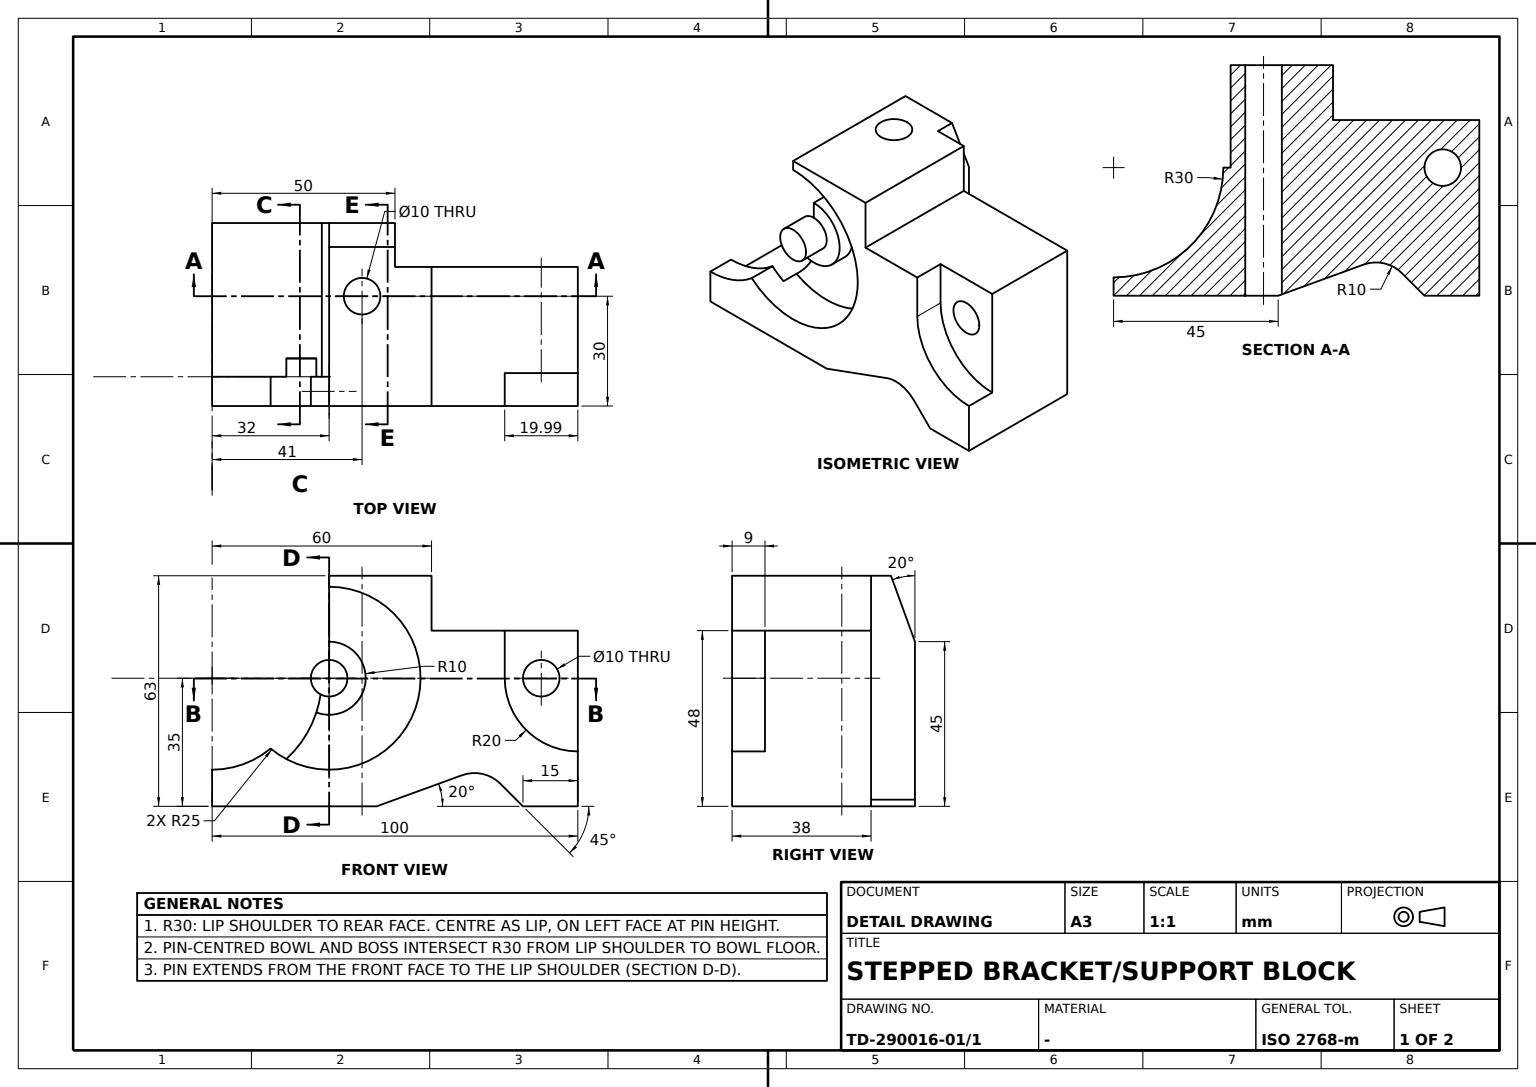
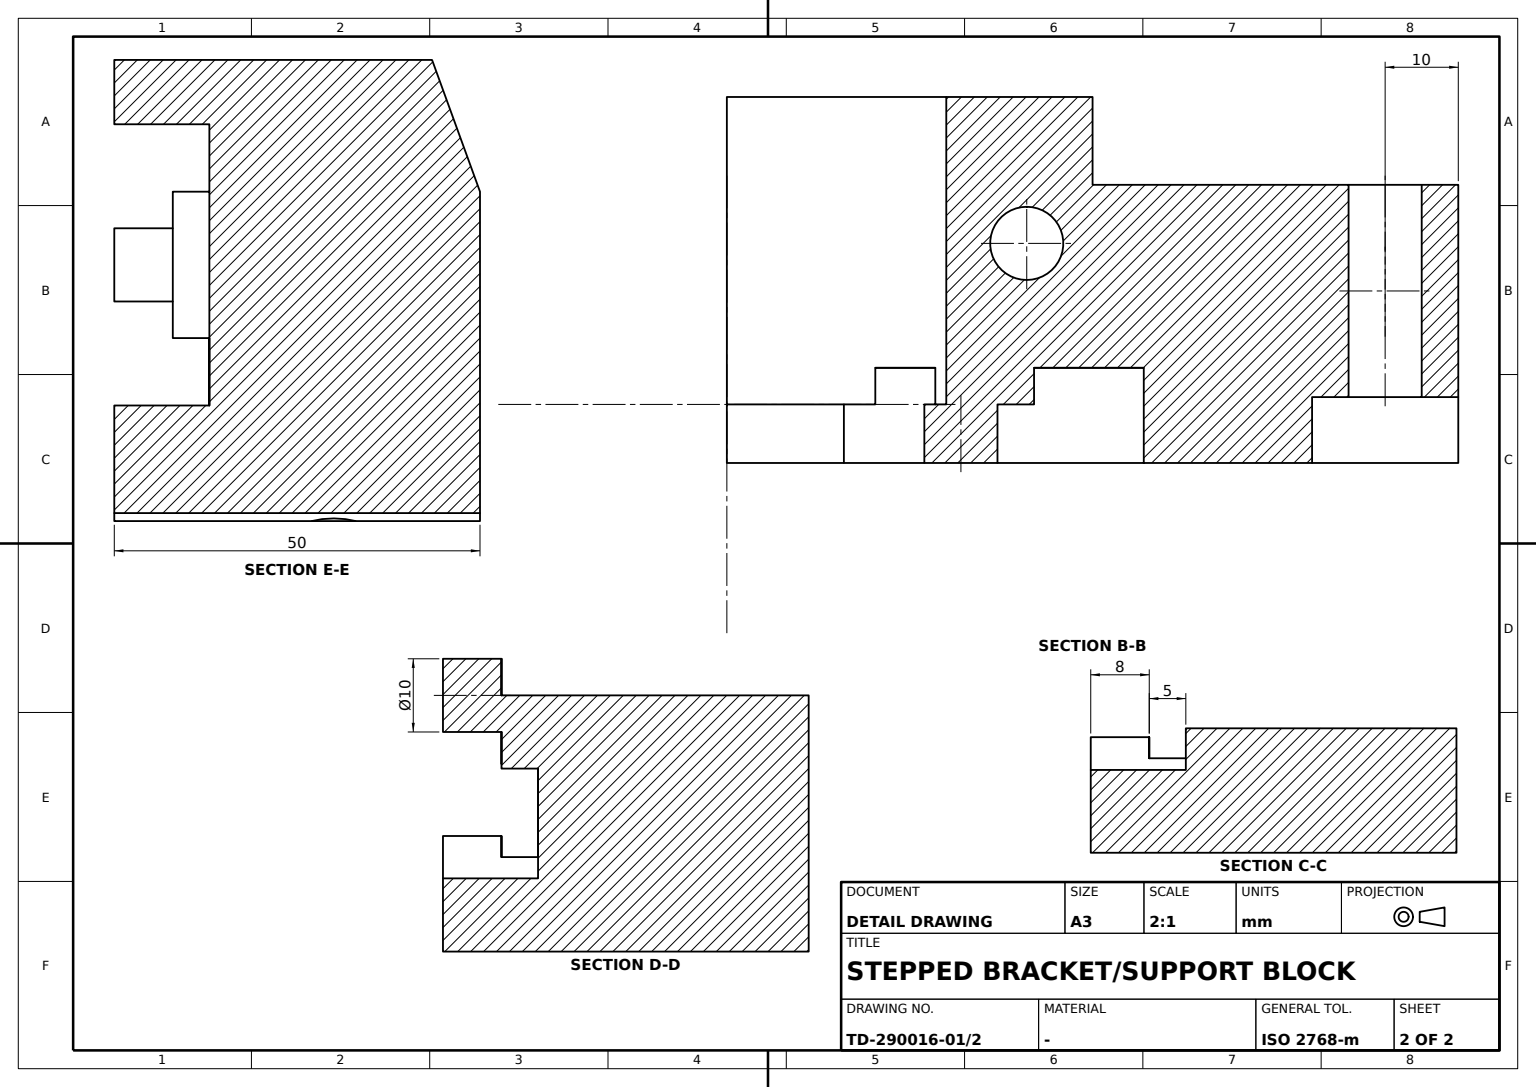
ISO-10303-21;
HEADER;
FILE_DESCRIPTION((''),'2;1');
FILE_NAME('','',(''),(''),'','','');
FILE_SCHEMA(('AUTOMOTIVE_DESIGN'));
ENDSEC;
DATA;
#1=APPLICATION_CONTEXT('');
#2=PRODUCT_CONTEXT('',#1,'mechanical');
#3=PRODUCT('','','',(#2));
#4=PRODUCT_DEFINITION_FORMATION('','',#3);
#5=PRODUCT_DEFINITION_CONTEXT('',#1,'design');
#6=PRODUCT_DEFINITION('','',#4,#5);
#7=PRODUCT_DEFINITION_SHAPE('','',#6);
#8=(LENGTH_UNIT()NAMED_UNIT(*)SI_UNIT(.MILLI.,.METRE.));
#9=(NAMED_UNIT(*)PLANE_ANGLE_UNIT()SI_UNIT($,.RADIAN.));
#10=(NAMED_UNIT(*)SI_UNIT($,.STERADIAN.)SOLID_ANGLE_UNIT());
#11=UNCERTAINTY_MEASURE_WITH_UNIT(LENGTH_MEASURE(1.E-05),#8,'distance_accuracy_value','');
#12=(GEOMETRIC_REPRESENTATION_CONTEXT(3)GLOBAL_UNCERTAINTY_ASSIGNED_CONTEXT((#11))GLOBAL_UNIT_ASSIGNED_CONTEXT((#8,#9,#10))REPRESENTATION_CONTEXT('',''));
#13=CARTESIAN_POINT('',(25.,78.83092,6.16908));
#14=VERTEX_POINT('',#13);
#15=CARTESIAN_POINT('',(-13.,78.83092,6.16908));
#16=VERTEX_POINT('',#15);
#17=CARTESIAN_POINT('',(6.,78.83092,6.16908));
#18=DIRECTION('',(-1.,0.,0.));
#19=VECTOR('',#18,1000.);
#20=LINE('',#17,#19);
#21=EDGE_CURVE('',#14,#16,#20,.T.);
#22=ORIENTED_EDGE('',*,*,#21,.F.);
#23=CARTESIAN_POINT('',(25.,68.339651,8.494938));
#24=VERTEX_POINT('',#23);
#25=CARTESIAN_POINT('',(25.,71.759852,-0.901988));
#26=DIRECTION('',(1.,0.,0.));
#27=DIRECTION('',(0.,1.,0.));
#28=AXIS2_PLACEMENT_3D('',#25,#26,#27);
#29=CIRCLE('',#28,10.);
#30=EDGE_CURVE('',#14,#24,#29,.T.);
#31=ORIENTED_EDGE('',*,*,#30,.T.);
#32=CARTESIAN_POINT('',(-13.,68.339651,8.494938));
#33=VERTEX_POINT('',#32);
#34=CARTESIAN_POINT('',(-0.66,68.339651,8.494938));
#35=LINE('',#34,#19);
#36=EDGE_CURVE('',#24,#33,#35,.T.);
#37=ORIENTED_EDGE('',*,*,#36,.T.);
#38=CARTESIAN_POINT('',(-13.,71.759852,-0.901988));
#39=AXIS2_PLACEMENT_3D('',#38,#18,#27);
#40=CIRCLE('',#39,10.);
#41=EDGE_CURVE('',#33,#16,#40,.T.);
#42=ORIENTED_EDGE('',*,*,#41,.T.);
#43=EDGE_LOOP('',(#22,#31,#37,#42));
#44=FACE_OUTER_BOUND('',#43,.T.);
#45=CARTESIAN_POINT('',(-0.66,71.759852,-0.901988));
#46=AXIS2_PLACEMENT_3D('',#45,#18,#27);
#47=CYLINDRICAL_SURFACE('',#46,10.);
#48=ADVANCED_FACE('',(#44),#47,.F.);
#49=CARTESIAN_POINT('',(17.,0.,5.));
#50=VERTEX_POINT('',#49);
#51=CARTESIAN_POINT('',(-25.,0.,5.));
#52=VERTEX_POINT('',#51);
#53=CARTESIAN_POINT('',(-4.,0.,5.));
#54=LINE('',#53,#19);
#55=EDGE_CURVE('',#50,#52,#54,.T.);
#56=ORIENTED_EDGE('',*,*,#55,.F.);
#57=CARTESIAN_POINT('',(17.,20.296875,12.908444));
#58=VERTEX_POINT('',#57);
#59=CARTESIAN_POINT('',(17.,0.,35.));
#60=AXIS2_PLACEMENT_3D('',#59,#26,#27);
#61=CIRCLE('',#60,30.);
#62=EDGE_CURVE('',#50,#58,#61,.T.);
#63=ORIENTED_EDGE('',*,*,#62,.T.);
#64=CARTESIAN_POINT('',(12.,20.296875,12.908444));
#65=VERTEX_POINT('',#64);
#66=CARTESIAN_POINT('',(3.34,20.296875,12.908444));
#67=LINE('',#66,#19);
#68=EDGE_CURVE('',#58,#65,#67,.T.);
#69=ORIENTED_EDGE('',*,*,#68,.T.);
#70=CARTESIAN_POINT('',(12.,28.5,25.632503));
#71=VERTEX_POINT('',#70);
#72=CARTESIAN_POINT('',(12.,0.,35.));
#73=AXIS2_PLACEMENT_3D('',#72,#26,#27);
#74=CIRCLE('',#73,30.);
#75=EDGE_CURVE('',#65,#71,#74,.T.);
#76=ORIENTED_EDGE('',*,*,#75,.T.);
#77=CARTESIAN_POINT('',(17.,28.5,25.632503));
#78=VERTEX_POINT('',#77);
#79=CARTESIAN_POINT('',(14.5,28.5,25.632503));
#80=VECTOR('',#26,1000.);
#81=LINE('',#79,#80);
#82=EDGE_CURVE('',#71,#78,#81,.T.);
#83=ORIENTED_EDGE('',*,*,#82,.T.);
#84=CARTESIAN_POINT('',(17.,29.671875,30.575089));
#85=VERTEX_POINT('',#84);
#86=EDGE_CURVE('',#78,#85,#61,.T.);
#87=ORIENTED_EDGE('',*,*,#86,.T.);
#88=CARTESIAN_POINT('',(17.,30.,35.));
#89=VERTEX_POINT('',#88);
#90=EDGE_CURVE('',#85,#89,#61,.T.);
#91=ORIENTED_EDGE('',*,*,#90,.T.);
#92=CARTESIAN_POINT('',(-25.,30.,35.));
#93=VERTEX_POINT('',#92);
#94=CARTESIAN_POINT('',(3.34,30.,35.));
#95=LINE('',#94,#19);
#96=EDGE_CURVE('',#89,#93,#95,.T.);
#97=ORIENTED_EDGE('',*,*,#96,.T.);
#98=CARTESIAN_POINT('',(-25.,0.,35.));
#99=AXIS2_PLACEMENT_3D('',#98,#26,#27);
#100=CIRCLE('',#99,30.);
#101=EDGE_CURVE('',#52,#93,#100,.T.);
#102=ORIENTED_EDGE('',*,*,#101,.F.);
#103=EDGE_LOOP('',(#56,#63,#69,#76,#83,#87,#91,#97,#102));
#104=FACE_OUTER_BOUND('',#103,.T.);
#105=CARTESIAN_POINT('',(-0.66,0.,35.));
#106=AXIS2_PLACEMENT_3D('',#105,#18,#27);
#107=CYLINDRICAL_SURFACE('',#106,30.);
#108=ADVANCED_FACE('',(#104),#107,.F.);
#109=CARTESIAN_POINT('',(25.,80.010269,35.));
#110=VERTEX_POINT('',#109);
#111=CARTESIAN_POINT('',(16.,80.010269,35.));
#112=VERTEX_POINT('',#111);
#113=CARTESIAN_POINT('',(20.5,80.010269,35.));
#114=LINE('',#113,#19);
#115=EDGE_CURVE('',#110,#112,#114,.T.);
#116=ORIENTED_EDGE('',*,*,#115,.F.);
#117=CARTESIAN_POINT('',(25.,100.,15.000003));
#118=VERTEX_POINT('',#117);
#119=CARTESIAN_POINT('',(25.,100.010269,35.));
#120=AXIS2_PLACEMENT_3D('',#119,#26,#27);
#121=CIRCLE('',#120,20.);
#122=EDGE_CURVE('',#110,#118,#121,.T.);
#123=ORIENTED_EDGE('',*,*,#122,.T.);
#124=CARTESIAN_POINT('',(16.,100.,15.000003));
#125=VERTEX_POINT('',#124);
#126=CARTESIAN_POINT('',(20.5,100.,15.000003));
#127=LINE('',#126,#19);
#128=EDGE_CURVE('',#118,#125,#127,.T.);
#129=ORIENTED_EDGE('',*,*,#128,.T.);
#130=CARTESIAN_POINT('',(16.,100.010269,35.));
#131=AXIS2_PLACEMENT_3D('',#130,#26,#27);
#132=CIRCLE('',#131,20.);
#133=EDGE_CURVE('',#112,#125,#132,.T.);
#134=ORIENTED_EDGE('',*,*,#133,.F.);
#135=EDGE_LOOP('',(#116,#123,#129,#134));
#136=FACE_OUTER_BOUND('',#135,.T.);
#137=CARTESIAN_POINT('',(20.5,100.010269,35.));
#138=AXIS2_PLACEMENT_3D('',#137,#18,#27);
#139=CYLINDRICAL_SURFACE('',#138,20.);
#140=ADVANCED_FACE('',(#136),#139,.F.);
#141=CARTESIAN_POINT('',(16.,95.,35.));
#142=VERTEX_POINT('',#141);
#143=CARTESIAN_POINT('',(-13.,95.,35.));
#144=VERTEX_POINT('',#143);
#145=CARTESIAN_POINT('',(-5.16,95.,35.));
#146=LINE('',#145,#19);
#147=EDGE_CURVE('',#142,#144,#146,.T.);
#148=ORIENTED_EDGE('',*,*,#147,.T.);
#149=CARTESIAN_POINT('',(-13.,85.,35.));
#150=VERTEX_POINT('',#149);
#151=CARTESIAN_POINT('',(-13.,90.,35.));
#152=AXIS2_PLACEMENT_3D('',#151,#18,#27);
#153=CIRCLE('',#152,5.);
#154=EDGE_CURVE('',#144,#150,#153,.T.);
#155=ORIENTED_EDGE('',*,*,#154,.T.);
#156=CARTESIAN_POINT('',(16.,85.,35.));
#157=VERTEX_POINT('',#156);
#158=CARTESIAN_POINT('',(-5.16,85.,35.));
#159=LINE('',#158,#19);
#160=EDGE_CURVE('',#157,#150,#159,.T.);
#161=ORIENTED_EDGE('',*,*,#160,.F.);
#162=CARTESIAN_POINT('',(16.,90.,35.));
#163=AXIS2_PLACEMENT_3D('',#162,#26,#27);
#164=CIRCLE('',#163,5.);
#165=EDGE_CURVE('',#157,#142,#164,.T.);
#166=ORIENTED_EDGE('',*,*,#165,.T.);
#167=EDGE_LOOP('',(#148,#155,#161,#166));
#168=FACE_OUTER_BOUND('',#167,.T.);
#169=CARTESIAN_POINT('',(-5.16,90.,35.));
#170=AXIS2_PLACEMENT_3D('',#169,#18,#27);
#171=CYLINDRICAL_SURFACE('',#170,5.);
#172=ADVANCED_FACE('',(#168),#171,.F.);
#173=ORIENTED_EDGE('',*,*,#101,.T.);
#174=CARTESIAN_POINT('',(-25.,32.,35.));
#175=VERTEX_POINT('',#174);
#176=CARTESIAN_POINT('',(-25.,31.,35.));
#177=VECTOR('',#27,1000.);
#178=LINE('',#176,#177);
#179=EDGE_CURVE('',#93,#175,#178,.T.);
#180=ORIENTED_EDGE('',*,*,#179,.T.);
#181=CARTESIAN_POINT('',(-25.,32.,45.));
#182=VERTEX_POINT('',#181);
#183=CARTESIAN_POINT('',(-25.,32.,40.));
#184=DIRECTION('',(0.,0.,-1.));
#185=VECTOR('',#184,1000.);
#186=LINE('',#183,#185);
#187=EDGE_CURVE('',#182,#175,#186,.T.);
#188=ORIENTED_EDGE('',*,*,#187,.F.);
#189=CARTESIAN_POINT('',(-25.,50.,45.));
#190=VERTEX_POINT('',#189);
#191=CARTESIAN_POINT('',(-25.,41.,45.));
#192=LINE('',#191,#177);
#193=EDGE_CURVE('',#182,#190,#192,.T.);
#194=ORIENTED_EDGE('',*,*,#193,.T.);
#195=CARTESIAN_POINT('',(-25.,50.,1.819851));
#196=VERTEX_POINT('',#195);
#197=CARTESIAN_POINT('',(-25.,50.,23.409926));
#198=LINE('',#197,#185);
#199=EDGE_CURVE('',#190,#196,#198,.T.);
#200=ORIENTED_EDGE('',*,*,#199,.T.);
#201=CARTESIAN_POINT('',(-25.,45.,0.));
#202=VERTEX_POINT('',#201);
#203=CARTESIAN_POINT('',(-25.,47.5,0.909926));
#204=DIRECTION('',(0.,0.939692621,0.342020143));
#205=VECTOR('',#204,1000.);
#206=LINE('',#203,#205);
#207=EDGE_CURVE('',#202,#196,#206,.T.);
#208=ORIENTED_EDGE('',*,*,#207,.F.);
#209=CARTESIAN_POINT('',(-25.,0.,0.));
#210=VERTEX_POINT('',#209);
#211=CARTESIAN_POINT('',(-25.,22.5,0.));
#212=LINE('',#211,#177);
#213=EDGE_CURVE('',#210,#202,#212,.T.);
#214=ORIENTED_EDGE('',*,*,#213,.F.);
#215=CARTESIAN_POINT('',(-25.,0.,2.5));
#216=LINE('',#215,#185);
#217=EDGE_CURVE('',#52,#210,#216,.T.);
#218=ORIENTED_EDGE('',*,*,#217,.F.);
#219=EDGE_LOOP('',(#173,#180,#188,#194,#200,#208,#214,#218));
#220=FACE_OUTER_BOUND('',#219,.T.);
#221=AXIS2_PLACEMENT_3D('',#209,#26,#27);
#222=PLANE('',#221);
#223=ADVANCED_FACE('',(#220),#222,.F.);
#224=CARTESIAN_POINT('',(25.,16.,15.790627));
#225=VERTEX_POINT('',#224);
#226=CARTESIAN_POINT('',(17.,16.,15.790627));
#227=VERTEX_POINT('',#226);
#228=CARTESIAN_POINT('',(22.5,16.,15.790627));
#229=LINE('',#228,#19);
#230=EDGE_CURVE('',#225,#227,#229,.T.);
#231=ORIENTED_EDGE('',*,*,#230,.T.);
#232=CARTESIAN_POINT('',(17.,0.,10.));
#233=VERTEX_POINT('',#232);
#234=AXIS2_PLACEMENT_3D('',#59,#18,#27);
#235=CIRCLE('',#234,25.);
#236=EDGE_CURVE('',#227,#233,#235,.T.);
#237=ORIENTED_EDGE('',*,*,#236,.T.);
#238=CARTESIAN_POINT('',(25.,0.,10.));
#239=VERTEX_POINT('',#238);
#240=CARTESIAN_POINT('',(21.,0.,10.));
#241=LINE('',#240,#19);
#242=EDGE_CURVE('',#239,#233,#241,.T.);
#243=ORIENTED_EDGE('',*,*,#242,.F.);
#244=CARTESIAN_POINT('',(25.,0.,35.));
#245=AXIS2_PLACEMENT_3D('',#244,#18,#27);
#246=CIRCLE('',#245,25.);
#247=EDGE_CURVE('',#225,#239,#246,.T.);
#248=ORIENTED_EDGE('',*,*,#247,.F.);
#249=EDGE_LOOP('',(#231,#237,#243,#248));
#250=FACE_OUTER_BOUND('',#249,.T.);
#251=CARTESIAN_POINT('',(21.,0.,35.));
#252=AXIS2_PLACEMENT_3D('',#251,#18,#27);
#253=CYLINDRICAL_SURFACE('',#252,25.);
#254=ADVANCED_FACE('',(#250),#253,.F.);
#255=CARTESIAN_POINT('',(12.,32.,45.));
#256=VERTEX_POINT('',#255);
#257=CARTESIAN_POINT('',(12.,32.,60.));
#258=VERTEX_POINT('',#257);
#259=CARTESIAN_POINT('',(12.,32.,52.5));
#260=DIRECTION('',(0.,0.,1.));
#261=VECTOR('',#260,1000.);
#262=LINE('',#259,#261);
#263=EDGE_CURVE('',#256,#258,#262,.T.);
#264=ORIENTED_EDGE('',*,*,#263,.F.);
#265=CARTESIAN_POINT('',(12.,42.,35.));
#266=VERTEX_POINT('',#265);
#267=CARTESIAN_POINT('',(12.,32.,35.));
#268=AXIS2_PLACEMENT_3D('',#267,#26,#27);
#269=CIRCLE('',#268,10.);
#270=EDGE_CURVE('',#266,#256,#269,.T.);
#271=ORIENTED_EDGE('',*,*,#270,.F.);
#272=EDGE_CURVE('',#71,#266,#269,.T.);
#273=ORIENTED_EDGE('',*,*,#272,.F.);
#274=ORIENTED_EDGE('',*,*,#75,.F.);
#275=CARTESIAN_POINT('',(12.,57.,35.));
#276=VERTEX_POINT('',#275);
#277=CIRCLE('',#268,25.);
#278=EDGE_CURVE('',#65,#276,#277,.T.);
#279=ORIENTED_EDGE('',*,*,#278,.T.);
#280=EDGE_CURVE('',#276,#258,#277,.T.);
#281=ORIENTED_EDGE('',*,*,#280,.T.);
#282=EDGE_LOOP('',(#264,#271,#273,#274,#279,#281));
#283=FACE_OUTER_BOUND('',#282,.T.);
#284=CARTESIAN_POINT('',(12.,0.,0.));
#285=AXIS2_PLACEMENT_3D('',#284,#26,#27);
#286=PLANE('',#285);
#287=ADVANCED_FACE('',(#283),#286,.T.);
#288=CARTESIAN_POINT('',(25.,37.,35.));
#289=VERTEX_POINT('',#288);
#290=CARTESIAN_POINT('',(25.,27.,35.));
#291=VERTEX_POINT('',#290);
#292=CARTESIAN_POINT('',(25.,32.,35.));
#293=AXIS2_PLACEMENT_3D('',#292,#26,#27);
#294=CIRCLE('',#293,5.);
#295=EDGE_CURVE('',#289,#291,#294,.T.);
#296=ORIENTED_EDGE('',*,*,#295,.T.);
#297=EDGE_CURVE('',#291,#289,#294,.T.);
#298=ORIENTED_EDGE('',*,*,#297,.T.);
#299=EDGE_LOOP('',(#296,#298));
#300=FACE_OUTER_BOUND('',#299,.T.);
#301=CARTESIAN_POINT('',(25.,0.,0.));
#302=AXIS2_PLACEMENT_3D('',#301,#26,#27);
#303=PLANE('',#302);
#304=ADVANCED_FACE('',(#300),#303,.T.);
#305=ORIENTED_EDGE('',*,*,#280,.F.);
#306=CARTESIAN_POINT('',(25.,57.,35.));
#307=VERTEX_POINT('',#306);
#308=CARTESIAN_POINT('',(22.5,57.,35.));
#309=LINE('',#308,#19);
#310=EDGE_CURVE('',#307,#276,#309,.T.);
#311=ORIENTED_EDGE('',*,*,#310,.F.);
#312=CARTESIAN_POINT('',(25.,32.,60.));
#313=VERTEX_POINT('',#312);
#314=CIRCLE('',#293,25.);
#315=EDGE_CURVE('',#307,#313,#314,.T.);
#316=ORIENTED_EDGE('',*,*,#315,.T.);
#317=CARTESIAN_POINT('',(18.5,32.,60.));
#318=LINE('',#317,#80);
#319=EDGE_CURVE('',#258,#313,#318,.T.);
#320=ORIENTED_EDGE('',*,*,#319,.F.);
#321=EDGE_LOOP('',(#305,#311,#316,#320));
#322=FACE_OUTER_BOUND('',#321,.T.);
#323=CARTESIAN_POINT('',(18.5,32.,35.));
#324=AXIS2_PLACEMENT_3D('',#323,#18,#27);
#325=CYLINDRICAL_SURFACE('',#324,25.);
#326=ADVANCED_FACE('',(#322),#325,.F.);
#327=CARTESIAN_POINT('',(-18.448536,32.,63.));
#328=VERTEX_POINT('',#327);
#329=CARTESIAN_POINT('',(-18.448536,50.,63.));
#330=VERTEX_POINT('',#329);
#331=CARTESIAN_POINT('',(-18.448536,41.,63.));
#332=LINE('',#331,#177);
#333=EDGE_CURVE('',#328,#330,#332,.T.);
#334=ORIENTED_EDGE('',*,*,#333,.T.);
#335=CARTESIAN_POINT('',(-21.724268,50.,54.));
#336=DIRECTION('',(0.342020143,0.,0.939692621));
#337=VECTOR('',#336,1000.);
#338=LINE('',#335,#337);
#339=EDGE_CURVE('',#190,#330,#338,.T.);
#340=ORIENTED_EDGE('',*,*,#339,.F.);
#341=ORIENTED_EDGE('',*,*,#193,.F.);
#342=CARTESIAN_POINT('',(-21.724268,32.,54.));
#343=LINE('',#342,#337);
#344=EDGE_CURVE('',#182,#328,#343,.T.);
#345=ORIENTED_EDGE('',*,*,#344,.T.);
#346=EDGE_LOOP('',(#334,#340,#341,#345));
#347=FACE_OUTER_BOUND('',#346,.T.);
#348=DIRECTION('',(-0.939692621,0.,0.342020143));
#349=AXIS2_PLACEMENT_3D('',#181,#348,#336);
#350=PLANE('',#349);
#351=ADVANCED_FACE('',(#347),#350,.T.);
#352=CARTESIAN_POINT('',(17.,42.,35.));
#353=VERTEX_POINT('',#352);
#354=CARTESIAN_POINT('',(14.5,42.,35.));
#355=LINE('',#354,#80);
#356=EDGE_CURVE('',#266,#353,#355,.T.);
#357=ORIENTED_EDGE('',*,*,#356,.F.);
#358=ORIENTED_EDGE('',*,*,#270,.T.);
#359=CARTESIAN_POINT('',(17.,32.,45.));
#360=VERTEX_POINT('',#359);
#361=CARTESIAN_POINT('',(14.5,32.,45.));
#362=LINE('',#361,#80);
#363=EDGE_CURVE('',#256,#360,#362,.T.);
#364=ORIENTED_EDGE('',*,*,#363,.T.);
#365=CARTESIAN_POINT('',(17.,32.,35.));
#366=AXIS2_PLACEMENT_3D('',#365,#26,#27);
#367=CIRCLE('',#366,10.);
#368=EDGE_CURVE('',#353,#360,#367,.T.);
#369=ORIENTED_EDGE('',*,*,#368,.F.);
#370=EDGE_LOOP('',(#357,#358,#364,#369));
#371=FACE_OUTER_BOUND('',#370,.T.);
#372=CARTESIAN_POINT('',(14.5,32.,35.));
#373=AXIS2_PLACEMENT_3D('',#372,#18,#27);
#374=CYLINDRICAL_SURFACE('',#373,10.);
#375=ADVANCED_FACE('',(#371),#374,.T.);
#376=CARTESIAN_POINT('',(16.,100.,48.));
#377=VERTEX_POINT('',#376);
#378=CARTESIAN_POINT('',(-13.,100.,48.));
#379=VERTEX_POINT('',#378);
#380=CARTESIAN_POINT('',(1.5,100.,48.));
#381=LINE('',#380,#19);
#382=EDGE_CURVE('',#377,#379,#381,.T.);
#383=ORIENTED_EDGE('',*,*,#382,.F.);
#384=CARTESIAN_POINT('',(16.,100.,31.5));
#385=LINE('',#384,#185);
#386=EDGE_CURVE('',#377,#125,#385,.T.);
#387=ORIENTED_EDGE('',*,*,#386,.T.);
#388=ORIENTED_EDGE('',*,*,#128,.F.);
#389=CARTESIAN_POINT('',(25.,100.,0.));
#390=VERTEX_POINT('',#389);
#391=CARTESIAN_POINT('',(25.,100.,7.500001));
#392=LINE('',#391,#261);
#393=EDGE_CURVE('',#390,#118,#392,.T.);
#394=ORIENTED_EDGE('',*,*,#393,.F.);
#395=CARTESIAN_POINT('',(-13.,100.,0.));
#396=VERTEX_POINT('',#395);
#397=CARTESIAN_POINT('',(6.,100.,0.));
#398=LINE('',#397,#80);
#399=EDGE_CURVE('',#396,#390,#398,.T.);
#400=ORIENTED_EDGE('',*,*,#399,.F.);
#401=CARTESIAN_POINT('',(-13.,100.,24.));
#402=LINE('',#401,#185);
#403=EDGE_CURVE('',#379,#396,#402,.T.);
#404=ORIENTED_EDGE('',*,*,#403,.F.);
#405=EDGE_LOOP('',(#383,#387,#388,#394,#400,#404));
#406=FACE_OUTER_BOUND('',#405,.T.);
#407=CARTESIAN_POINT('',(0.,100.,63.));
#408=DIRECTION('',(0.,-1.,0.));
#409=AXIS2_PLACEMENT_3D('',#407,#408,#184);
#410=PLANE('',#409);
#411=ADVANCED_FACE('',(#406),#410,.F.);
#412=ORIENTED_EDGE('',*,*,#199,.F.);
#413=ORIENTED_EDGE('',*,*,#339,.T.);
#414=CARTESIAN_POINT('',(-13.,50.,63.));
#415=VERTEX_POINT('',#414);
#416=CARTESIAN_POINT('',(-15.724268,50.,63.));
#417=LINE('',#416,#80);
#418=EDGE_CURVE('',#330,#415,#417,.T.);
#419=ORIENTED_EDGE('',*,*,#418,.T.);
#420=CARTESIAN_POINT('',(-13.,50.,1.819851));
#421=VERTEX_POINT('',#420);
#422=CARTESIAN_POINT('',(-13.,50.,32.409926));
#423=LINE('',#422,#185);
#424=EDGE_CURVE('',#415,#421,#423,.T.);
#425=ORIENTED_EDGE('',*,*,#424,.T.);
#426=CARTESIAN_POINT('',(-19.,50.,1.819851));
#427=LINE('',#426,#19);
#428=EDGE_CURVE('',#421,#196,#427,.T.);
#429=ORIENTED_EDGE('',*,*,#428,.T.);
#430=EDGE_LOOP('',(#412,#413,#419,#425,#429));
#431=FACE_OUTER_BOUND('',#430,.T.);
#432=AXIS2_PLACEMENT_3D('',#414,#408,#18);
#433=PLANE('',#432);
#434=ADVANCED_FACE('',(#431),#433,.F.);
#435=CARTESIAN_POINT('',(25.,85.,0.));
#436=VERTEX_POINT('',#435);
#437=CARTESIAN_POINT('',(25.,81.91546,3.08454));
#438=DIRECTION('',(0.,-0.707106781,0.707106781));
#439=VECTOR('',#438,1000.);
#440=LINE('',#437,#439);
#441=EDGE_CURVE('',#436,#14,#440,.T.);
#442=ORIENTED_EDGE('',*,*,#441,.T.);
#443=ORIENTED_EDGE('',*,*,#21,.T.);
#444=CARTESIAN_POINT('',(-13.,85.,0.));
#445=VERTEX_POINT('',#444);
#446=CARTESIAN_POINT('',(-13.,81.91546,3.08454));
#447=LINE('',#446,#439);
#448=EDGE_CURVE('',#445,#16,#447,.T.);
#449=ORIENTED_EDGE('',*,*,#448,.F.);
#450=CARTESIAN_POINT('',(6.,85.,0.));
#451=LINE('',#450,#19);
#452=EDGE_CURVE('',#436,#445,#451,.T.);
#453=ORIENTED_EDGE('',*,*,#452,.F.);
#454=EDGE_LOOP('',(#442,#443,#449,#453));
#455=FACE_OUTER_BOUND('',#454,.T.);
#456=DIRECTION('',(0.,-0.707106781,-0.707106781));
#457=AXIS2_PLACEMENT_3D('',#435,#456,#438);
#458=PLANE('',#457);
#459=ADVANCED_FACE('',(#455),#458,.T.);
#460=VERTEX_POINT('',#301);
#461=CARTESIAN_POINT('',(0.,0.,0.));
#462=LINE('',#461,#80);
#463=EDGE_CURVE('',#210,#460,#462,.T.);
#464=ORIENTED_EDGE('',*,*,#463,.F.);
#465=ORIENTED_EDGE('',*,*,#213,.T.);
#466=CARTESIAN_POINT('',(-8.,45.,0.));
#467=VERTEX_POINT('',#466);
#468=CARTESIAN_POINT('',(-16.5,45.,0.));
#469=LINE('',#468,#19);
#470=EDGE_CURVE('',#467,#202,#469,.T.);
#471=ORIENTED_EDGE('',*,*,#470,.F.);
#472=CARTESIAN_POINT('',(-10.,41.,0.));
#473=VERTEX_POINT('',#472);
#474=CARTESIAN_POINT('',(-5.,41.,0.));
#475=AXIS2_PLACEMENT_3D('',#474,#184,#27);
#476=CIRCLE('',#475,5.);
#477=EDGE_CURVE('',#473,#467,#476,.T.);
#478=ORIENTED_EDGE('',*,*,#477,.F.);
#479=CARTESIAN_POINT('',(0.,41.,0.));
#480=VERTEX_POINT('',#479);
#481=EDGE_CURVE('',#480,#473,#476,.T.);
#482=ORIENTED_EDGE('',*,*,#481,.F.);
#483=CARTESIAN_POINT('',(-2.,45.,0.));
#484=VERTEX_POINT('',#483);
#485=EDGE_CURVE('',#484,#480,#476,.T.);
#486=ORIENTED_EDGE('',*,*,#485,.F.);
#487=CARTESIAN_POINT('',(25.,45.,0.));
#488=VERTEX_POINT('',#487);
#489=CARTESIAN_POINT('',(11.5,45.,0.));
#490=LINE('',#489,#19);
#491=EDGE_CURVE('',#488,#484,#490,.T.);
#492=ORIENTED_EDGE('',*,*,#491,.F.);
#493=CARTESIAN_POINT('',(25.,22.5,0.));
#494=LINE('',#493,#177);
#495=EDGE_CURVE('',#460,#488,#494,.T.);
#496=ORIENTED_EDGE('',*,*,#495,.F.);
#497=EDGE_LOOP('',(#464,#465,#471,#478,#482,#486,#492,#496));
#498=FACE_OUTER_BOUND('',#497,.T.);
#499=AXIS2_PLACEMENT_3D('',#461,#184,#27);
#500=PLANE('',#499);
#501=ADVANCED_FACE('',(#498),#500,.T.);
#502=VERTEX_POINT('',#365);
#503=CARTESIAN_POINT('',(17.,32.,40.));
#504=VERTEX_POINT('',#503);
#505=CARTESIAN_POINT('',(17.,32.,37.5));
#506=LINE('',#505,#261);
#507=EDGE_CURVE('',#502,#504,#506,.T.);
#508=ORIENTED_EDGE('',*,*,#507,.F.);
#509=CARTESIAN_POINT('',(17.,31.,35.));
#510=LINE('',#509,#177);
#511=EDGE_CURVE('',#89,#502,#510,.T.);
#512=ORIENTED_EDGE('',*,*,#511,.F.);
#513=ORIENTED_EDGE('',*,*,#90,.F.);
#514=CARTESIAN_POINT('',(17.,27.,35.));
#515=VERTEX_POINT('',#514);
#516=CIRCLE('',#366,5.);
#517=EDGE_CURVE('',#515,#85,#516,.T.);
#518=ORIENTED_EDGE('',*,*,#517,.F.);
#519=EDGE_CURVE('',#504,#515,#516,.T.);
#520=ORIENTED_EDGE('',*,*,#519,.F.);
#521=EDGE_LOOP('',(#508,#512,#513,#518,#520));
#522=FACE_OUTER_BOUND('',#521,.T.);
#523=CARTESIAN_POINT('',(17.,0.,0.));
#524=AXIS2_PLACEMENT_3D('',#523,#26,#27);
#525=PLANE('',#524);
#526=ADVANCED_FACE('',(#522),#525,.F.);
#527=ORIENTED_EDGE('',*,*,#315,.F.);
#528=EDGE_CURVE('',#225,#307,#314,.T.);
#529=ORIENTED_EDGE('',*,*,#528,.F.);
#530=ORIENTED_EDGE('',*,*,#247,.T.);
#531=CARTESIAN_POINT('',(25.,0.,5.));
#532=LINE('',#531,#185);
#533=EDGE_CURVE('',#239,#460,#532,.T.);
#534=ORIENTED_EDGE('',*,*,#533,.T.);
#535=ORIENTED_EDGE('',*,*,#495,.T.);
#536=CARTESIAN_POINT('',(25.,56.669825,4.247469));
#537=DIRECTION('',(0.,-0.939692621,-0.342020143));
#538=VECTOR('',#537,1000.);
#539=LINE('',#536,#538);
#540=EDGE_CURVE('',#24,#488,#539,.T.);
#541=ORIENTED_EDGE('',*,*,#540,.F.);
#542=ORIENTED_EDGE('',*,*,#30,.F.);
#543=ORIENTED_EDGE('',*,*,#441,.F.);
#544=CARTESIAN_POINT('',(25.,92.5,0.));
#545=LINE('',#544,#177);
#546=EDGE_CURVE('',#436,#390,#545,.T.);
#547=ORIENTED_EDGE('',*,*,#546,.T.);
#548=ORIENTED_EDGE('',*,*,#393,.T.);
#549=ORIENTED_EDGE('',*,*,#122,.F.);
#550=CARTESIAN_POINT('',(25.,80.010269,48.));
#551=VERTEX_POINT('',#550);
#552=CARTESIAN_POINT('',(25.,80.010269,41.5));
#553=LINE('',#552,#185);
#554=EDGE_CURVE('',#551,#110,#553,.T.);
#555=ORIENTED_EDGE('',*,*,#554,.F.);
#556=CARTESIAN_POINT('',(25.,60.,48.));
#557=VERTEX_POINT('',#556);
#558=CARTESIAN_POINT('',(25.,70.005135,48.));
#559=LINE('',#558,#177);
#560=EDGE_CURVE('',#557,#551,#559,.T.);
#561=ORIENTED_EDGE('',*,*,#560,.F.);
#562=CARTESIAN_POINT('',(25.,60.,63.));
#563=VERTEX_POINT('',#562);
#564=CARTESIAN_POINT('',(25.,60.,55.5));
#565=LINE('',#564,#185);
#566=EDGE_CURVE('',#563,#557,#565,.T.);
#567=ORIENTED_EDGE('',*,*,#566,.F.);
#568=CARTESIAN_POINT('',(25.,32.,63.));
#569=VERTEX_POINT('',#568);
#570=CARTESIAN_POINT('',(25.,46.,63.));
#571=VECTOR('',#408,1000.);
#572=LINE('',#570,#571);
#573=EDGE_CURVE('',#563,#569,#572,.T.);
#574=ORIENTED_EDGE('',*,*,#573,.T.);
#575=CARTESIAN_POINT('',(25.,32.,61.5));
#576=LINE('',#575,#185);
#577=EDGE_CURVE('',#569,#313,#576,.T.);
#578=ORIENTED_EDGE('',*,*,#577,.T.);
#579=EDGE_LOOP('',(#527,#529,#530,#534,#535,#541,#542,#543,#547,#548,#549,#555,#561,#567,#574,#578));
#580=FACE_OUTER_BOUND('',#579,.T.);
#581=ADVANCED_FACE('',(#580),#303,.T.);
#582=ORIENTED_EDGE('',*,*,#147,.F.);
#583=EDGE_CURVE('',#142,#157,#164,.T.);
#584=ORIENTED_EDGE('',*,*,#583,.T.);
#585=ORIENTED_EDGE('',*,*,#160,.T.);
#586=EDGE_CURVE('',#150,#144,#153,.T.);
#587=ORIENTED_EDGE('',*,*,#586,.T.);
#588=EDGE_LOOP('',(#582,#584,#585,#587));
#589=FACE_OUTER_BOUND('',#588,.T.);
#590=ADVANCED_FACE('',(#589),#171,.F.);
#591=CARTESIAN_POINT('',(-13.,59.169825,5.157395));
#592=LINE('',#591,#538);
#593=EDGE_CURVE('',#33,#421,#592,.T.);
#594=ORIENTED_EDGE('',*,*,#593,.T.);
#595=ORIENTED_EDGE('',*,*,#424,.F.);
#596=CARTESIAN_POINT('',(-13.,60.,63.));
#597=VERTEX_POINT('',#596);
#598=CARTESIAN_POINT('',(-13.,55.,63.));
#599=LINE('',#598,#177);
#600=EDGE_CURVE('',#415,#597,#599,.T.);
#601=ORIENTED_EDGE('',*,*,#600,.T.);
#602=CARTESIAN_POINT('',(-13.,60.,48.));
#603=VERTEX_POINT('',#602);
#604=CARTESIAN_POINT('',(-13.,60.,55.5));
#605=LINE('',#604,#185);
#606=EDGE_CURVE('',#597,#603,#605,.T.);
#607=ORIENTED_EDGE('',*,*,#606,.T.);
#608=CARTESIAN_POINT('',(-13.,80.,48.));
#609=LINE('',#608,#571);
#610=EDGE_CURVE('',#379,#603,#609,.T.);
#611=ORIENTED_EDGE('',*,*,#610,.F.);
#612=ORIENTED_EDGE('',*,*,#403,.T.);
#613=CARTESIAN_POINT('',(-13.,92.5,0.));
#614=LINE('',#613,#571);
#615=EDGE_CURVE('',#396,#445,#614,.T.);
#616=ORIENTED_EDGE('',*,*,#615,.T.);
#617=ORIENTED_EDGE('',*,*,#448,.T.);
#618=ORIENTED_EDGE('',*,*,#41,.F.);
#619=EDGE_LOOP('',(#594,#595,#601,#607,#611,#612,#616,#617,#618));
#620=FACE_OUTER_BOUND('',#619,.T.);
#621=ORIENTED_EDGE('',*,*,#586,.F.);
#622=ORIENTED_EDGE('',*,*,#154,.F.);
#623=EDGE_LOOP('',(#621,#622));
#624=FACE_BOUND('',#623,.T.);
#625=AXIS2_PLACEMENT_3D('',#414,#18,#27);
#626=PLANE('',#625);
#627=ADVANCED_FACE('',(#620,#624),#626,.T.);
#628=CARTESIAN_POINT('',(6.,60.,48.));
#629=LINE('',#628,#19);
#630=EDGE_CURVE('',#557,#603,#629,.T.);
#631=ORIENTED_EDGE('',*,*,#630,.T.);
#632=ORIENTED_EDGE('',*,*,#606,.F.);
#633=CARTESIAN_POINT('',(6.,60.,63.));
#634=LINE('',#633,#19);
#635=EDGE_CURVE('',#563,#597,#634,.T.);
#636=ORIENTED_EDGE('',*,*,#635,.F.);
#637=ORIENTED_EDGE('',*,*,#566,.T.);
#638=EDGE_LOOP('',(#631,#632,#636,#637));
#639=FACE_OUTER_BOUND('',#638,.T.);
#640=AXIS2_PLACEMENT_3D('',#562,#27,#184);
#641=PLANE('',#640);
#642=ADVANCED_FACE('',(#639),#641,.T.);
#643=ORIENTED_EDGE('',*,*,#428,.F.);
#644=ORIENTED_EDGE('',*,*,#593,.F.);
#645=ORIENTED_EDGE('',*,*,#36,.F.);
#646=ORIENTED_EDGE('',*,*,#540,.T.);
#647=ORIENTED_EDGE('',*,*,#491,.T.);
#648=CARTESIAN_POINT('',(-2.33587,45.251902,0.091685));
#649=CARTESIAN_POINT('',(-2.700319,45.470157,0.171123));
#650=CARTESIAN_POINT('',(-3.088999,45.650083,0.236611));
#651=CARTESIAN_POINT('',(-3.89134,45.92126,0.335311));
#652=CARTESIAN_POINT('',(-4.737269,46.019433,0.371043));
#653=CARTESIAN_POINT('',(-5.15821,46.023826,0.372642));
#654=CARTESIAN_POINT('',(-5.997161,45.944129,0.343635));
#655=CARTESIAN_POINT('',(-6.797352,45.694,0.252595));
#656=CARTESIAN_POINT('',(-7.182476,45.52736,0.191943));
#657=CARTESIAN_POINT('',(-7.571179,45.308743,0.112373));
#658=CARTESIAN_POINT('',(-7.929492,45.052081,0.018956));
#659=CARTESIAN_POINT('',(-7.953134,45.034883,0.012696));
#660=CARTESIAN_POINT('',(-7.976636,45.017523,0.006378));
#661=B_SPLINE_CURVE_WITH_KNOTS('',5,(#483,#648,#649,#650,#651,#652,#653,#654,#655,#656,#657,#658,#659,#660,#466),.UNSPECIFIED.,.F.,.F.,(6,3,3,3,6),(0.,3.038663349,5.990909473,8.965280824,9.176658544),.UNSPECIFIED.);
#662=EDGE_CURVE('',#484,#467,#661,.T.);
#663=ORIENTED_EDGE('',*,*,#662,.T.);
#664=ORIENTED_EDGE('',*,*,#470,.T.);
#665=ORIENTED_EDGE('',*,*,#207,.T.);
#666=EDGE_LOOP('',(#643,#644,#645,#646,#647,#663,#664,#665));
#667=FACE_OUTER_BOUND('',#666,.T.);
#668=DIRECTION('',(0.,-0.342020143,0.939692621));
#669=AXIS2_PLACEMENT_3D('',#487,#668,#204);
#670=PLANE('',#669);
#671=ADVANCED_FACE('',(#667),#670,.F.);
#672=CARTESIAN_POINT('',(-10.,41.,63.));
#673=VERTEX_POINT('',#672);
#674=CARTESIAN_POINT('',(-10.,41.,30.84));
#675=LINE('',#674,#185);
#676=EDGE_CURVE('',#673,#473,#675,.T.);
#677=ORIENTED_EDGE('',*,*,#676,.F.);
#678=CARTESIAN_POINT('',(0.,41.,63.));
#679=VERTEX_POINT('',#678);
#680=CARTESIAN_POINT('',(-5.,41.,63.));
#681=AXIS2_PLACEMENT_3D('',#680,#260,#26);
#682=CIRCLE('',#681,5.);
#683=EDGE_CURVE('',#673,#679,#682,.T.);
#684=ORIENTED_EDGE('',*,*,#683,.T.);
#685=CARTESIAN_POINT('',(0.,41.,30.84));
#686=LINE('',#685,#185);
#687=EDGE_CURVE('',#679,#480,#686,.T.);
#688=ORIENTED_EDGE('',*,*,#687,.T.);
#689=ORIENTED_EDGE('',*,*,#481,.T.);
#690=EDGE_LOOP('',(#677,#684,#688,#689));
#691=FACE_OUTER_BOUND('',#690,.T.);
#692=CARTESIAN_POINT('',(-5.,41.,30.84));
#693=AXIS2_PLACEMENT_3D('',#692,#184,#26);
#694=CYLINDRICAL_SURFACE('',#693,5.);
#695=ADVANCED_FACE('',(#691),#694,.F.);
#696=EDGE_CURVE('',#78,#353,#367,.T.);
#697=ORIENTED_EDGE('',*,*,#696,.F.);
#698=ORIENTED_EDGE('',*,*,#82,.F.);
#699=ORIENTED_EDGE('',*,*,#272,.T.);
#700=ORIENTED_EDGE('',*,*,#356,.T.);
#701=EDGE_LOOP('',(#697,#698,#699,#700));
#702=FACE_OUTER_BOUND('',#701,.T.);
#703=ADVANCED_FACE('',(#702),#374,.T.);
#704=ORIENTED_EDGE('',*,*,#452,.T.);
#705=ORIENTED_EDGE('',*,*,#615,.F.);
#706=ORIENTED_EDGE('',*,*,#399,.T.);
#707=ORIENTED_EDGE('',*,*,#546,.F.);
#708=EDGE_LOOP('',(#704,#705,#706,#707));
#709=FACE_OUTER_BOUND('',#708,.T.);
#710=ADVANCED_FACE('',(#709),#500,.T.);
#711=ORIENTED_EDGE('',*,*,#68,.F.);
#712=AXIS2_PLACEMENT_3D('',#365,#18,#27);
#713=CIRCLE('',#712,25.);
#714=EDGE_CURVE('',#58,#227,#713,.T.);
#715=ORIENTED_EDGE('',*,*,#714,.T.);
#716=ORIENTED_EDGE('',*,*,#230,.F.);
#717=ORIENTED_EDGE('',*,*,#528,.T.);
#718=ORIENTED_EDGE('',*,*,#310,.T.);
#719=ORIENTED_EDGE('',*,*,#278,.F.);
#720=EDGE_LOOP('',(#711,#715,#716,#717,#718,#719));
#721=FACE_OUTER_BOUND('',#720,.T.);
#722=ADVANCED_FACE('',(#721),#325,.F.);
#723=ORIENTED_EDGE('',*,*,#635,.T.);
#724=ORIENTED_EDGE('',*,*,#600,.F.);
#725=ORIENTED_EDGE('',*,*,#418,.F.);
#726=ORIENTED_EDGE('',*,*,#333,.F.);
#727=CARTESIAN_POINT('',(3.275732,32.,63.));
#728=LINE('',#727,#19);
#729=EDGE_CURVE('',#569,#328,#728,.T.);
#730=ORIENTED_EDGE('',*,*,#729,.F.);
#731=ORIENTED_EDGE('',*,*,#573,.F.);
#732=EDGE_LOOP('',(#723,#724,#725,#726,#730,#731));
#733=FACE_OUTER_BOUND('',#732,.T.);
#734=EDGE_CURVE('',#679,#673,#682,.T.);
#735=ORIENTED_EDGE('',*,*,#734,.F.);
#736=ORIENTED_EDGE('',*,*,#683,.F.);
#737=EDGE_LOOP('',(#735,#736));
#738=FACE_BOUND('',#737,.T.);
#739=CARTESIAN_POINT('',(0.,0.,63.));
#740=AXIS2_PLACEMENT_3D('',#739,#184,#27);
#741=PLANE('',#740);
#742=ADVANCED_FACE('',(#733,#738),#741,.F.);
#743=ORIENTED_EDGE('',*,*,#165,.F.);
#744=ORIENTED_EDGE('',*,*,#583,.F.);
#745=EDGE_LOOP('',(#743,#744));
#746=FACE_BOUND('',#745,.T.);
#747=ORIENTED_EDGE('',*,*,#133,.T.);
#748=ORIENTED_EDGE('',*,*,#386,.F.);
#749=CARTESIAN_POINT('',(16.,80.010269,48.));
#750=VERTEX_POINT('',#749);
#751=CARTESIAN_POINT('',(16.,90.005135,48.));
#752=LINE('',#751,#571);
#753=EDGE_CURVE('',#377,#750,#752,.T.);
#754=ORIENTED_EDGE('',*,*,#753,.T.);
#755=CARTESIAN_POINT('',(16.,80.010269,41.5));
#756=LINE('',#755,#185);
#757=EDGE_CURVE('',#750,#112,#756,.T.);
#758=ORIENTED_EDGE('',*,*,#757,.T.);
#759=EDGE_LOOP('',(#747,#748,#754,#758));
#760=FACE_OUTER_BOUND('',#759,.T.);
#761=CARTESIAN_POINT('',(16.,0.,0.));
#762=AXIS2_PLACEMENT_3D('',#761,#26,#27);
#763=PLANE('',#762);
#764=ADVANCED_FACE('',(#746,#760),#763,.T.);
#765=ORIENTED_EDGE('',*,*,#115,.T.);
#766=ORIENTED_EDGE('',*,*,#757,.F.);
#767=CARTESIAN_POINT('',(20.5,80.010269,48.));
#768=LINE('',#767,#19);
#769=EDGE_CURVE('',#551,#750,#768,.T.);
#770=ORIENTED_EDGE('',*,*,#769,.F.);
#771=ORIENTED_EDGE('',*,*,#554,.T.);
#772=EDGE_LOOP('',(#765,#766,#770,#771));
#773=FACE_OUTER_BOUND('',#772,.T.);
#774=CARTESIAN_POINT('',(25.,80.010269,63.));
#775=AXIS2_PLACEMENT_3D('',#774,#27,#184);
#776=PLANE('',#775);
#777=ADVANCED_FACE('',(#773),#776,.T.);
#778=ORIENTED_EDGE('',*,*,#463,.T.);
#779=ORIENTED_EDGE('',*,*,#533,.F.);
#780=ORIENTED_EDGE('',*,*,#242,.T.);
#781=CARTESIAN_POINT('',(17.,0.,7.5));
#782=LINE('',#781,#185);
#783=EDGE_CURVE('',#233,#50,#782,.T.);
#784=ORIENTED_EDGE('',*,*,#783,.T.);
#785=ORIENTED_EDGE('',*,*,#55,.T.);
#786=ORIENTED_EDGE('',*,*,#217,.T.);
#787=EDGE_LOOP('',(#778,#779,#780,#784,#785,#786));
#788=FACE_OUTER_BOUND('',#787,.T.);
#789=AXIS2_PLACEMENT_3D('',#461,#27,#260);
#790=PLANE('',#789);
#791=ADVANCED_FACE('',(#788),#790,.F.);
#792=ORIENTED_EDGE('',*,*,#560,.T.);
#793=ORIENTED_EDGE('',*,*,#769,.T.);
#794=ORIENTED_EDGE('',*,*,#753,.F.);
#795=ORIENTED_EDGE('',*,*,#382,.T.);
#796=ORIENTED_EDGE('',*,*,#610,.T.);
#797=ORIENTED_EDGE('',*,*,#630,.F.);
#798=EDGE_LOOP('',(#792,#793,#794,#795,#796,#797));
#799=FACE_OUTER_BOUND('',#798,.T.);
#800=CARTESIAN_POINT('',(25.,100.,48.));
#801=AXIS2_PLACEMENT_3D('',#800,#184,#408);
#802=PLANE('',#801);
#803=ADVANCED_FACE('',(#799),#802,.F.);
#804=CARTESIAN_POINT('',(17.,37.,35.));
#805=VERTEX_POINT('',#804);
#806=EDGE_CURVE('',#805,#504,#516,.T.);
#807=ORIENTED_EDGE('',*,*,#806,.T.);
#808=ORIENTED_EDGE('',*,*,#519,.T.);
#809=CARTESIAN_POINT('',(21.,27.,35.));
#810=LINE('',#809,#80);
#811=EDGE_CURVE('',#515,#291,#810,.T.);
#812=ORIENTED_EDGE('',*,*,#811,.T.);
#813=ORIENTED_EDGE('',*,*,#295,.F.);
#814=CARTESIAN_POINT('',(21.,37.,35.));
#815=LINE('',#814,#80);
#816=EDGE_CURVE('',#805,#289,#815,.T.);
#817=ORIENTED_EDGE('',*,*,#816,.F.);
#818=EDGE_LOOP('',(#807,#808,#812,#813,#817));
#819=FACE_OUTER_BOUND('',#818,.T.);
#820=CARTESIAN_POINT('',(21.,32.,35.));
#821=AXIS2_PLACEMENT_3D('',#820,#18,#27);
#822=CYLINDRICAL_SURFACE('',#821,5.);
#823=ADVANCED_FACE('',(#819),#822,.T.);
#824=ORIENTED_EDGE('',*,*,#507,.T.);
#825=CARTESIAN_POINT('',(17.,32.,42.5));
#826=LINE('',#825,#261);
#827=EDGE_CURVE('',#504,#360,#826,.T.);
#828=ORIENTED_EDGE('',*,*,#827,.T.);
#829=ORIENTED_EDGE('',*,*,#363,.F.);
#830=ORIENTED_EDGE('',*,*,#263,.T.);
#831=ORIENTED_EDGE('',*,*,#319,.T.);
#832=ORIENTED_EDGE('',*,*,#577,.F.);
#833=ORIENTED_EDGE('',*,*,#729,.T.);
#834=ORIENTED_EDGE('',*,*,#344,.F.);
#835=ORIENTED_EDGE('',*,*,#187,.T.);
#836=CARTESIAN_POINT('',(-4.,32.,35.));
#837=LINE('',#836,#19);
#838=EDGE_CURVE('',#502,#175,#837,.T.);
#839=ORIENTED_EDGE('',*,*,#838,.F.);
#840=EDGE_LOOP('',(#824,#828,#829,#830,#831,#832,#833,#834,#835,#839));
#841=FACE_OUTER_BOUND('',#840,.T.);
#842=CARTESIAN_POINT('',(-33.369202,32.,63.));
#843=AXIS2_PLACEMENT_3D('',#842,#27,#26);
#844=PLANE('',#843);
#845=ADVANCED_FACE('',(#841),#844,.F.);
#846=ORIENTED_EDGE('',*,*,#687,.F.);
#847=ORIENTED_EDGE('',*,*,#734,.T.);
#848=ORIENTED_EDGE('',*,*,#676,.T.);
#849=ORIENTED_EDGE('',*,*,#477,.T.);
#850=ORIENTED_EDGE('',*,*,#662,.F.);
#851=ORIENTED_EDGE('',*,*,#485,.T.);
#852=EDGE_LOOP('',(#846,#847,#848,#849,#850,#851));
#853=FACE_OUTER_BOUND('',#852,.T.);
#854=ADVANCED_FACE('',(#853),#694,.F.);
#855=ORIENTED_EDGE('',*,*,#783,.F.);
#856=ORIENTED_EDGE('',*,*,#236,.F.);
#857=ORIENTED_EDGE('',*,*,#714,.F.);
#858=ORIENTED_EDGE('',*,*,#62,.F.);
#859=EDGE_LOOP('',(#855,#856,#857,#858));
#860=FACE_OUTER_BOUND('',#859,.T.);
#861=ADVANCED_FACE('',(#860),#525,.F.);
#862=ORIENTED_EDGE('',*,*,#838,.T.);
#863=ORIENTED_EDGE('',*,*,#179,.F.);
#864=ORIENTED_EDGE('',*,*,#96,.F.);
#865=ORIENTED_EDGE('',*,*,#511,.T.);
#866=EDGE_LOOP('',(#862,#863,#864,#865));
#867=FACE_OUTER_BOUND('',#866,.T.);
#868=CARTESIAN_POINT('',(0.,0.,35.));
#869=AXIS2_PLACEMENT_3D('',#868,#260,#26);
#870=PLANE('',#869);
#871=ADVANCED_FACE('',(#867),#870,.T.);
#872=ORIENTED_EDGE('',*,*,#811,.F.);
#873=ORIENTED_EDGE('',*,*,#517,.T.);
#874=EDGE_CURVE('',#85,#805,#516,.T.);
#875=ORIENTED_EDGE('',*,*,#874,.T.);
#876=ORIENTED_EDGE('',*,*,#816,.T.);
#877=ORIENTED_EDGE('',*,*,#297,.F.);
#878=EDGE_LOOP('',(#872,#873,#875,#876,#877));
#879=FACE_OUTER_BOUND('',#878,.T.);
#880=ADVANCED_FACE('',(#879),#822,.T.);
#881=ORIENTED_EDGE('',*,*,#806,.F.);
#882=ORIENTED_EDGE('',*,*,#874,.F.);
#883=ORIENTED_EDGE('',*,*,#86,.F.);
#884=ORIENTED_EDGE('',*,*,#696,.T.);
#885=ORIENTED_EDGE('',*,*,#368,.T.);
#886=ORIENTED_EDGE('',*,*,#827,.F.);
#887=EDGE_LOOP('',(#881,#882,#883,#884,#885,#886));
#888=FACE_OUTER_BOUND('',#887,.T.);
#889=ADVANCED_FACE('',(#888),#525,.T.);
#890=CLOSED_SHELL('',(#48,#108,#140,#172,#223,#254,#287,#304,#326,#351,#375,#411,#434,#459,#501,#526,#581,#590,#627,#642,#671,#695,#703,#710,#722,#742,#764,#777,#791,#803,#823,#845,#854,#861,#871,#880,#889));
#891=MANIFOLD_SOLID_BREP('',#890);
#892=ADVANCED_BREP_SHAPE_REPRESENTATION('',(#891),#12);
#893=SHAPE_DEFINITION_REPRESENTATION(#7,#892);
ENDSEC;
END-ISO-10303-21;
